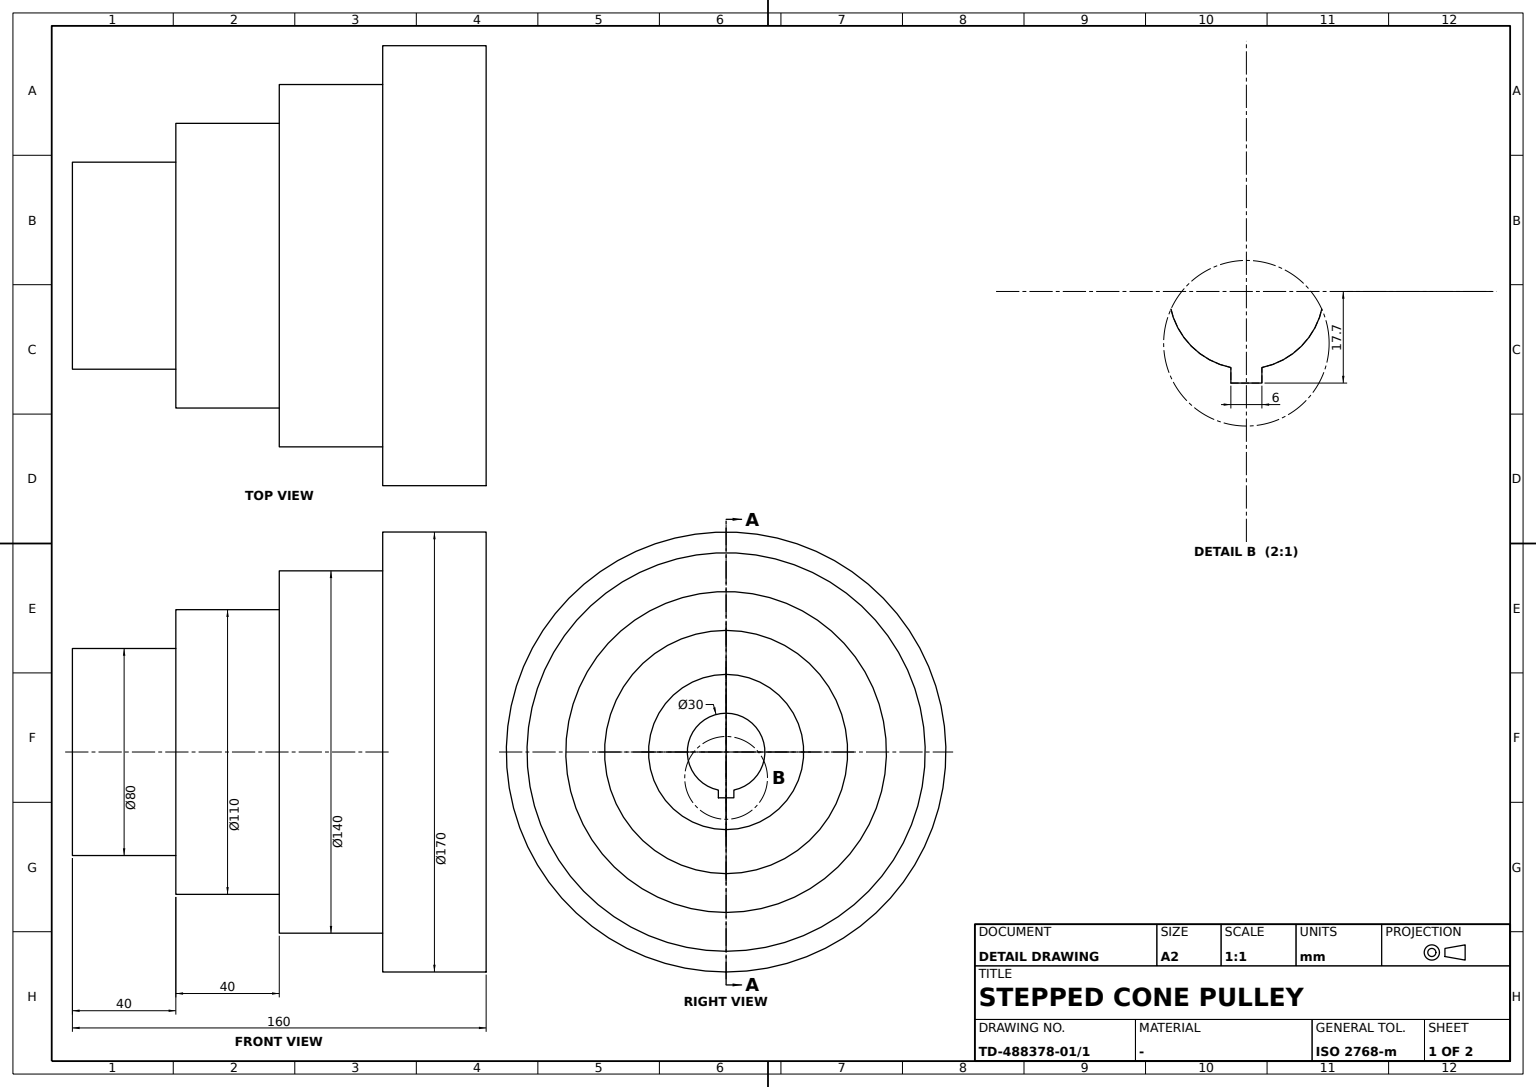
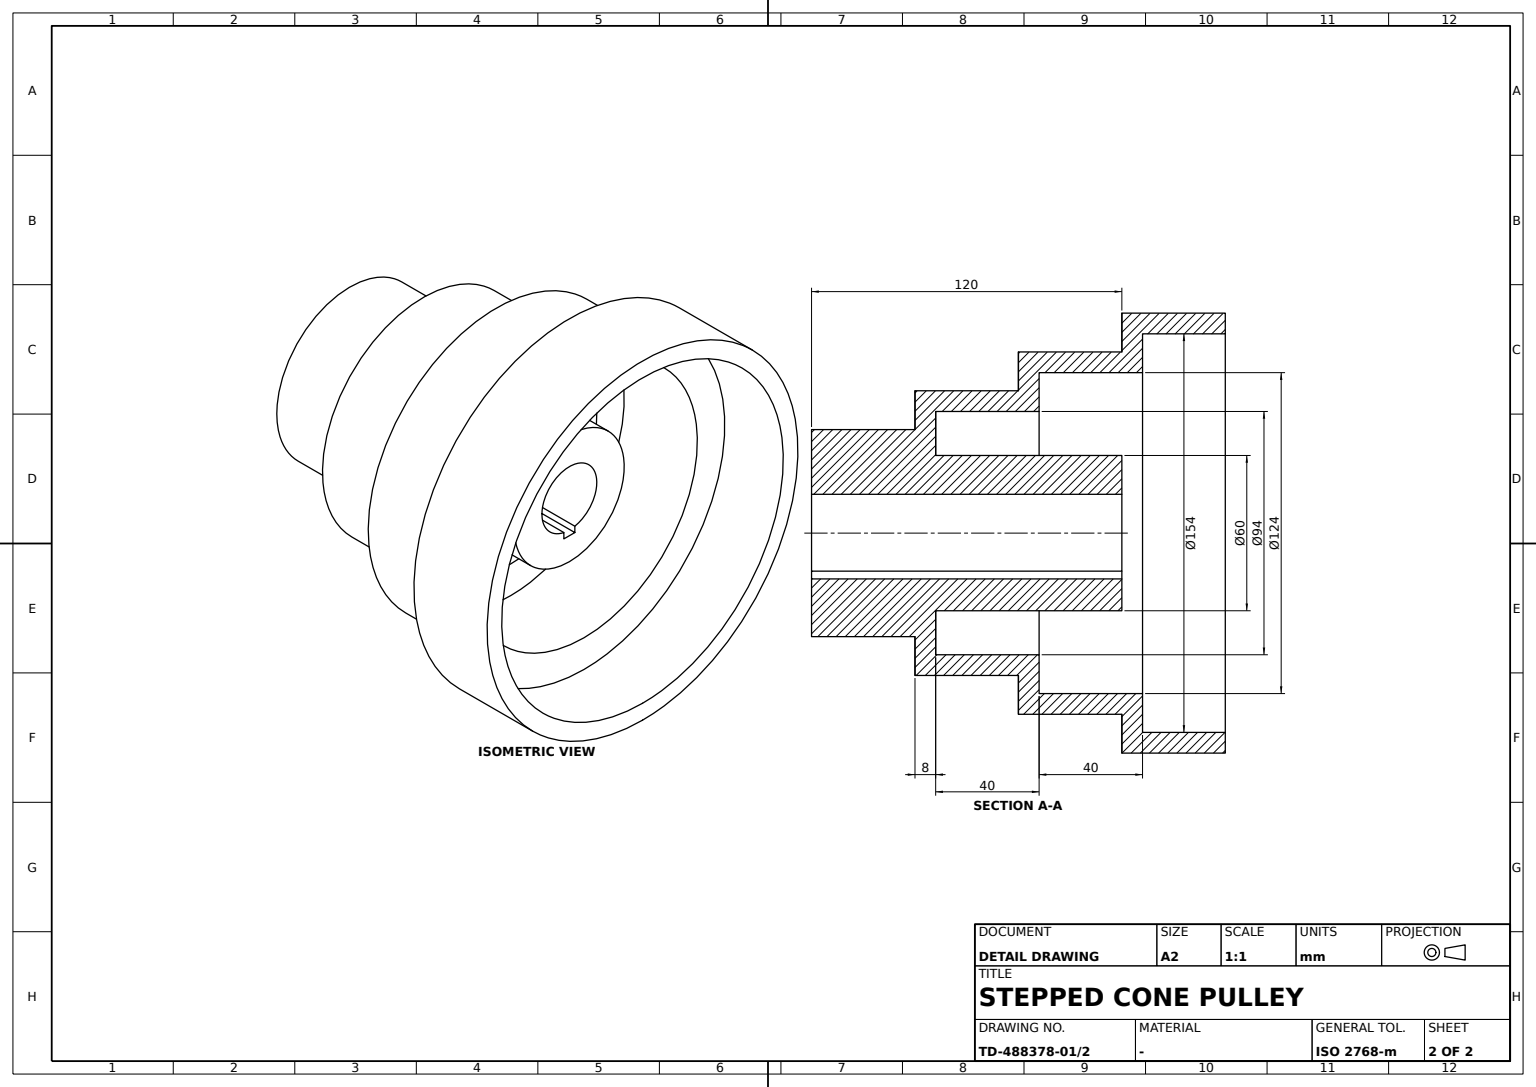
ISO-10303-21;
HEADER;
FILE_DESCRIPTION((''),'2;1');
FILE_NAME('','',(''),(''),'','','');
FILE_SCHEMA(('AUTOMOTIVE_DESIGN'));
ENDSEC;
DATA;
#1=APPLICATION_CONTEXT('');
#2=PRODUCT_CONTEXT('',#1,'mechanical');
#3=PRODUCT('','','',(#2));
#4=PRODUCT_DEFINITION_FORMATION('','',#3);
#5=PRODUCT_DEFINITION_CONTEXT('',#1,'design');
#6=PRODUCT_DEFINITION('','',#4,#5);
#7=PRODUCT_DEFINITION_SHAPE('','',#6);
#8=(LENGTH_UNIT()NAMED_UNIT(*)SI_UNIT(.MILLI.,.METRE.));
#9=(NAMED_UNIT(*)PLANE_ANGLE_UNIT()SI_UNIT($,.RADIAN.));
#10=(NAMED_UNIT(*)SI_UNIT($,.STERADIAN.)SOLID_ANGLE_UNIT());
#11=UNCERTAINTY_MEASURE_WITH_UNIT(LENGTH_MEASURE(0.005),#8,'distance_accuracy_value','');
#12=(GEOMETRIC_REPRESENTATION_CONTEXT(3)GLOBAL_UNCERTAINTY_ASSIGNED_CONTEXT((#11))GLOBAL_UNIT_ASSIGNED_CONTEXT((#8,#9,#10))REPRESENTATION_CONTEXT('',''));
#13=CARTESIAN_POINT('',(0.,80.,-70.));
#14=VERTEX_POINT('',#13);
#15=CARTESIAN_POINT('',(0.,80.,0.));
#16=DIRECTION('',(0.,-1.,0.));
#17=DIRECTION('',(0.,0.,-1.));
#18=AXIS2_PLACEMENT_3D('',#15,#16,#17);
#19=CIRCLE('',#18,70.);
#20=EDGE_CURVE('',#14,#14,#19,.T.);
#21=ORIENTED_EDGE('',*,*,#20,.T.);
#22=EDGE_LOOP('',(#21));
#23=FACE_BOUND('',#22,.T.);
#24=CARTESIAN_POINT('',(0.,80.,-55.));
#25=VERTEX_POINT('',#24);
#26=CIRCLE('',#18,55.);
#27=EDGE_CURVE('',#25,#25,#26,.T.);
#28=ORIENTED_EDGE('',*,*,#27,.F.);
#29=EDGE_LOOP('',(#28));
#30=FACE_BOUND('',#29,.T.);
#31=CARTESIAN_POINT('',(0.,80.,70.));
#32=DIRECTION('',(1.,0.,0.));
#33=AXIS2_PLACEMENT_3D('',#31,#16,#32);
#34=PLANE('',#33);
#35=ADVANCED_FACE('',(#23,#30),#34,.T.);
#36=CARTESIAN_POINT('',(0.,48.,-30.));
#37=VERTEX_POINT('',#36);
#38=CARTESIAN_POINT('',(0.,48.,0.));
#39=AXIS2_PLACEMENT_3D('',#38,#16,#17);
#40=CIRCLE('',#39,30.);
#41=EDGE_CURVE('',#37,#37,#40,.T.);
#42=ORIENTED_EDGE('',*,*,#41,.T.);
#43=EDGE_LOOP('',(#42));
#44=FACE_BOUND('',#43,.T.);
#45=CARTESIAN_POINT('',(0.,48.,-47.));
#46=VERTEX_POINT('',#45);
#47=CIRCLE('',#39,47.);
#48=EDGE_CURVE('',#46,#46,#47,.T.);
#49=ORIENTED_EDGE('',*,*,#48,.F.);
#50=EDGE_LOOP('',(#49));
#51=FACE_BOUND('',#50,.T.);
#52=CARTESIAN_POINT('',(0.,48.,30.));
#53=AXIS2_PLACEMENT_3D('',#52,#16,#32);
#54=PLANE('',#53);
#55=ADVANCED_FACE('',(#44,#51),#54,.F.);
#56=CARTESIAN_POINT('',(0.,160.,-85.));
#57=VERTEX_POINT('',#56);
#58=CARTESIAN_POINT('',(0.,160.,0.));
#59=AXIS2_PLACEMENT_3D('',#58,#16,#17);
#60=CIRCLE('',#59,85.);
#61=EDGE_CURVE('',#57,#57,#60,.T.);
#62=ORIENTED_EDGE('',*,*,#61,.F.);
#63=EDGE_LOOP('',(#62));
#64=FACE_BOUND('',#63,.T.);
#65=CARTESIAN_POINT('',(0.,160.,-77.));
#66=VERTEX_POINT('',#65);
#67=CIRCLE('',#59,77.);
#68=EDGE_CURVE('',#66,#66,#67,.T.);
#69=ORIENTED_EDGE('',*,*,#68,.T.);
#70=EDGE_LOOP('',(#69));
#71=FACE_BOUND('',#70,.T.);
#72=CARTESIAN_POINT('',(0.,160.,77.));
#73=AXIS2_PLACEMENT_3D('',#72,#16,#32);
#74=PLANE('',#73);
#75=ADVANCED_FACE('',(#64,#71),#74,.F.);
#76=CARTESIAN_POINT('',(3.,120.,-14.696938));
#77=VERTEX_POINT('',#76);
#78=CARTESIAN_POINT('',(3.,120.,-17.696938));
#79=VERTEX_POINT('',#78);
#80=VECTOR('',#17,1000.);
#81=LINE('',#76,#80);
#82=EDGE_CURVE('',#77,#79,#81,.T.);
#83=ORIENTED_EDGE('',*,*,#82,.F.);
#84=CARTESIAN_POINT('',(-3.,120.,-14.696938));
#85=VERTEX_POINT('',#84);
#86=CARTESIAN_POINT('',(0.,120.,0.));
#87=AXIS2_PLACEMENT_3D('',#86,#16,#17);
#88=CIRCLE('',#87,15.);
#89=EDGE_CURVE('',#77,#85,#88,.T.);
#90=ORIENTED_EDGE('',*,*,#89,.T.);
#91=CARTESIAN_POINT('',(-3.,120.,-17.696938));
#92=VERTEX_POINT('',#91);
#93=DIRECTION('',(0.,0.,1.));
#94=VECTOR('',#93,1000.);
#95=LINE('',#91,#94);
#96=EDGE_CURVE('',#92,#85,#95,.T.);
#97=ORIENTED_EDGE('',*,*,#96,.F.);
#98=DIRECTION('',(-1.,0.,0.));
#99=VECTOR('',#98,1000.);
#100=LINE('',#78,#99);
#101=EDGE_CURVE('',#79,#92,#100,.T.);
#102=ORIENTED_EDGE('',*,*,#101,.F.);
#103=EDGE_LOOP('',(#83,#90,#97,#102));
#104=FACE_BOUND('',#103,.T.);
#105=CARTESIAN_POINT('',(0.,120.,-30.));
#106=VERTEX_POINT('',#105);
#107=CIRCLE('',#87,30.);
#108=EDGE_CURVE('',#106,#106,#107,.T.);
#109=ORIENTED_EDGE('',*,*,#108,.F.);
#110=EDGE_LOOP('',(#109));
#111=FACE_BOUND('',#110,.T.);
#112=CARTESIAN_POINT('',(0.,120.,15.));
#113=AXIS2_PLACEMENT_3D('',#112,#16,#32);
#114=PLANE('',#113);
#115=ADVANCED_FACE('',(#104,#111),#114,.F.);
#116=CARTESIAN_POINT('',(0.,88.,-47.));
#117=VERTEX_POINT('',#116);
#118=CARTESIAN_POINT('',(0.,88.,0.));
#119=AXIS2_PLACEMENT_3D('',#118,#16,#17);
#120=CIRCLE('',#119,47.);
#121=EDGE_CURVE('',#117,#117,#120,.T.);
#122=ORIENTED_EDGE('',*,*,#121,.T.);
#123=EDGE_LOOP('',(#122));
#124=FACE_BOUND('',#123,.T.);
#125=CARTESIAN_POINT('',(0.,88.,-62.));
#126=VERTEX_POINT('',#125);
#127=CIRCLE('',#119,62.);
#128=EDGE_CURVE('',#126,#126,#127,.T.);
#129=ORIENTED_EDGE('',*,*,#128,.F.);
#130=EDGE_LOOP('',(#129));
#131=FACE_BOUND('',#130,.T.);
#132=CARTESIAN_POINT('',(0.,88.,47.));
#133=AXIS2_PLACEMENT_3D('',#132,#16,#32);
#134=PLANE('',#133);
#135=ADVANCED_FACE('',(#124,#131),#134,.F.);
#136=CARTESIAN_POINT('',(0.,40.,-40.));
#137=VERTEX_POINT('',#136);
#138=CARTESIAN_POINT('',(0.,40.,0.));
#139=AXIS2_PLACEMENT_3D('',#138,#16,#17);
#140=CIRCLE('',#139,40.);
#141=EDGE_CURVE('',#137,#137,#140,.T.);
#142=ORIENTED_EDGE('',*,*,#141,.T.);
#143=EDGE_LOOP('',(#142));
#144=FACE_BOUND('',#143,.T.);
#145=CARTESIAN_POINT('',(0.,0.,-40.));
#146=VERTEX_POINT('',#145);
#147=CARTESIAN_POINT('',(0.,0.,0.));
#148=AXIS2_PLACEMENT_3D('',#147,#16,#17);
#149=CIRCLE('',#148,40.);
#150=EDGE_CURVE('',#146,#146,#149,.T.);
#151=ORIENTED_EDGE('',*,*,#150,.F.);
#152=EDGE_LOOP('',(#151));
#153=FACE_BOUND('',#152,.T.);
#154=AXIS2_PLACEMENT_3D('',#15,#16,#32);
#155=CYLINDRICAL_SURFACE('',#154,40.);
#156=ADVANCED_FACE('',(#144,#153),#155,.T.);
#157=CARTESIAN_POINT('',(-3.,0.,-14.696938));
#158=VERTEX_POINT('',#157);
#159=VECTOR('',#16,1000.);
#160=LINE('',#157,#159);
#161=EDGE_CURVE('',#158,#85,#160,.F.);
#162=ORIENTED_EDGE('',*,*,#161,.F.);
#163=CARTESIAN_POINT('',(-3.,0.,-17.696938));
#164=VERTEX_POINT('',#163);
#165=LINE('',#163,#94);
#166=EDGE_CURVE('',#164,#158,#165,.T.);
#167=ORIENTED_EDGE('',*,*,#166,.F.);
#168=DIRECTION('',(0.,1.,0.));
#169=VECTOR('',#168,1000.);
#170=LINE('',#163,#169);
#171=EDGE_CURVE('',#164,#92,#170,.T.);
#172=ORIENTED_EDGE('',*,*,#171,.T.);
#173=ORIENTED_EDGE('',*,*,#96,.T.);
#174=EDGE_LOOP('',(#162,#167,#172,#173));
#175=FACE_BOUND('',#174,.T.);
#176=AXIS2_PLACEMENT_3D('',#163,#98,#93);
#177=PLANE('',#176);
#178=ADVANCED_FACE('',(#175),#177,.F.);
#179=ORIENTED_EDGE('',*,*,#82,.T.);
#180=CARTESIAN_POINT('',(3.,0.,-17.696938));
#181=VERTEX_POINT('',#180);
#182=LINE('',#180,#169);
#183=EDGE_CURVE('',#181,#79,#182,.T.);
#184=ORIENTED_EDGE('',*,*,#183,.F.);
#185=CARTESIAN_POINT('',(3.,0.,-14.696938));
#186=VERTEX_POINT('',#185);
#187=LINE('',#185,#80);
#188=EDGE_CURVE('',#186,#181,#187,.T.);
#189=ORIENTED_EDGE('',*,*,#188,.F.);
#190=LINE('',#185,#159);
#191=EDGE_CURVE('',#186,#77,#190,.F.);
#192=ORIENTED_EDGE('',*,*,#191,.T.);
#193=EDGE_LOOP('',(#179,#184,#189,#192));
#194=FACE_BOUND('',#193,.T.);
#195=AXIS2_PLACEMENT_3D('',#185,#32,#17);
#196=PLANE('',#195);
#197=ADVANCED_FACE('',(#194),#196,.F.);
#198=CARTESIAN_POINT('',(0.,128.,-77.));
#199=VERTEX_POINT('',#198);
#200=CARTESIAN_POINT('',(0.,128.,0.));
#201=AXIS2_PLACEMENT_3D('',#200,#16,#17);
#202=CIRCLE('',#201,77.);
#203=EDGE_CURVE('',#199,#199,#202,.T.);
#204=ORIENTED_EDGE('',*,*,#203,.T.);
#205=EDGE_LOOP('',(#204));
#206=FACE_BOUND('',#205,.T.);
#207=ORIENTED_EDGE('',*,*,#68,.F.);
#208=EDGE_LOOP('',(#207));
#209=FACE_BOUND('',#208,.T.);
#210=CYLINDRICAL_SURFACE('',#154,77.);
#211=ADVANCED_FACE('',(#206,#209),#210,.F.);
#212=ORIENTED_EDGE('',*,*,#128,.T.);
#213=EDGE_LOOP('',(#212));
#214=FACE_BOUND('',#213,.T.);
#215=CARTESIAN_POINT('',(0.,128.,-62.));
#216=VERTEX_POINT('',#215);
#217=CIRCLE('',#201,62.);
#218=EDGE_CURVE('',#216,#216,#217,.T.);
#219=ORIENTED_EDGE('',*,*,#218,.F.);
#220=EDGE_LOOP('',(#219));
#221=FACE_BOUND('',#220,.T.);
#222=CYLINDRICAL_SURFACE('',#154,62.);
#223=ADVANCED_FACE('',(#214,#221),#222,.F.);
#224=CARTESIAN_POINT('',(0.,40.,-55.));
#225=VERTEX_POINT('',#224);
#226=CIRCLE('',#139,55.);
#227=EDGE_CURVE('',#225,#225,#226,.T.);
#228=ORIENTED_EDGE('',*,*,#227,.T.);
#229=EDGE_LOOP('',(#228));
#230=FACE_BOUND('',#229,.T.);
#231=ORIENTED_EDGE('',*,*,#141,.F.);
#232=EDGE_LOOP('',(#231));
#233=FACE_BOUND('',#232,.T.);
#234=CARTESIAN_POINT('',(0.,40.,55.));
#235=AXIS2_PLACEMENT_3D('',#234,#16,#32);
#236=PLANE('',#235);
#237=ADVANCED_FACE('',(#230,#233),#236,.T.);
#238=ORIENTED_EDGE('',*,*,#61,.T.);
#239=EDGE_LOOP('',(#238));
#240=FACE_BOUND('',#239,.T.);
#241=CARTESIAN_POINT('',(0.,120.,-85.));
#242=VERTEX_POINT('',#241);
#243=CIRCLE('',#87,85.);
#244=EDGE_CURVE('',#242,#242,#243,.T.);
#245=ORIENTED_EDGE('',*,*,#244,.F.);
#246=EDGE_LOOP('',(#245));
#247=FACE_BOUND('',#246,.T.);
#248=CYLINDRICAL_SURFACE('',#154,85.);
#249=ADVANCED_FACE('',(#240,#247),#248,.T.);
#250=ORIENTED_EDGE('',*,*,#161,.T.);
#251=ORIENTED_EDGE('',*,*,#89,.F.);
#252=ORIENTED_EDGE('',*,*,#191,.F.);
#253=CIRCLE('',#148,15.);
#254=EDGE_CURVE('',#186,#158,#253,.T.);
#255=ORIENTED_EDGE('',*,*,#254,.T.);
#256=EDGE_LOOP('',(#250,#251,#252,#255));
#257=FACE_BOUND('',#256,.T.);
#258=CYLINDRICAL_SURFACE('',#154,15.);
#259=ADVANCED_FACE('',(#257),#258,.F.);
#260=ORIENTED_EDGE('',*,*,#227,.F.);
#261=EDGE_LOOP('',(#260));
#262=FACE_BOUND('',#261,.T.);
#263=ORIENTED_EDGE('',*,*,#27,.T.);
#264=EDGE_LOOP('',(#263));
#265=FACE_BOUND('',#264,.T.);
#266=CYLINDRICAL_SURFACE('',#154,55.);
#267=ADVANCED_FACE('',(#262,#265),#266,.T.);
#268=ORIENTED_EDGE('',*,*,#218,.T.);
#269=EDGE_LOOP('',(#268));
#270=FACE_BOUND('',#269,.T.);
#271=ORIENTED_EDGE('',*,*,#203,.F.);
#272=EDGE_LOOP('',(#271));
#273=FACE_BOUND('',#272,.T.);
#274=CARTESIAN_POINT('',(0.,128.,62.));
#275=AXIS2_PLACEMENT_3D('',#274,#16,#32);
#276=PLANE('',#275);
#277=ADVANCED_FACE('',(#270,#273),#276,.F.);
#278=ORIENTED_EDGE('',*,*,#101,.T.);
#279=ORIENTED_EDGE('',*,*,#171,.F.);
#280=LINE('',#180,#99);
#281=EDGE_CURVE('',#181,#164,#280,.T.);
#282=ORIENTED_EDGE('',*,*,#281,.F.);
#283=ORIENTED_EDGE('',*,*,#183,.T.);
#284=EDGE_LOOP('',(#278,#279,#282,#283));
#285=FACE_BOUND('',#284,.T.);
#286=AXIS2_PLACEMENT_3D('',#180,#17,#98);
#287=PLANE('',#286);
#288=ADVANCED_FACE('',(#285),#287,.F.);
#289=ORIENTED_EDGE('',*,*,#41,.F.);
#290=EDGE_LOOP('',(#289));
#291=FACE_BOUND('',#290,.T.);
#292=ORIENTED_EDGE('',*,*,#108,.T.);
#293=EDGE_LOOP('',(#292));
#294=FACE_BOUND('',#293,.T.);
#295=CYLINDRICAL_SURFACE('',#154,30.);
#296=ADVANCED_FACE('',(#291,#294),#295,.T.);
#297=CARTESIAN_POINT('',(0.,120.,-70.));
#298=VERTEX_POINT('',#297);
#299=CIRCLE('',#87,70.);
#300=EDGE_CURVE('',#298,#298,#299,.T.);
#301=ORIENTED_EDGE('',*,*,#300,.F.);
#302=EDGE_LOOP('',(#301));
#303=FACE_BOUND('',#302,.T.);
#304=ORIENTED_EDGE('',*,*,#244,.T.);
#305=EDGE_LOOP('',(#304));
#306=FACE_BOUND('',#305,.T.);
#307=ADVANCED_FACE('',(#303,#306),#114,.T.);
#308=ORIENTED_EDGE('',*,*,#20,.F.);
#309=EDGE_LOOP('',(#308));
#310=FACE_BOUND('',#309,.T.);
#311=ORIENTED_EDGE('',*,*,#300,.T.);
#312=EDGE_LOOP('',(#311));
#313=FACE_BOUND('',#312,.T.);
#314=CYLINDRICAL_SURFACE('',#154,70.);
#315=ADVANCED_FACE('',(#310,#313),#314,.T.);
#316=ORIENTED_EDGE('',*,*,#48,.T.);
#317=EDGE_LOOP('',(#316));
#318=FACE_BOUND('',#317,.T.);
#319=ORIENTED_EDGE('',*,*,#121,.F.);
#320=EDGE_LOOP('',(#319));
#321=FACE_BOUND('',#320,.T.);
#322=CYLINDRICAL_SURFACE('',#154,47.);
#323=ADVANCED_FACE('',(#318,#321),#322,.F.);
#324=ORIENTED_EDGE('',*,*,#166,.T.);
#325=ORIENTED_EDGE('',*,*,#254,.F.);
#326=ORIENTED_EDGE('',*,*,#188,.T.);
#327=ORIENTED_EDGE('',*,*,#281,.T.);
#328=EDGE_LOOP('',(#324,#325,#326,#327));
#329=FACE_BOUND('',#328,.T.);
#330=ORIENTED_EDGE('',*,*,#150,.T.);
#331=EDGE_LOOP('',(#330));
#332=FACE_BOUND('',#331,.T.);
#333=CARTESIAN_POINT('',(0.,0.,40.));
#334=AXIS2_PLACEMENT_3D('',#333,#16,#32);
#335=PLANE('',#334);
#336=ADVANCED_FACE('',(#329,#332),#335,.T.);
#337=CLOSED_SHELL('',(#35,#55,#75,#115,#135,#156,#178,#197,#211,#223,#237,#249,#259,#267,#277,#288,#296,#307,#315,#323,#336));
#338=MANIFOLD_SOLID_BREP('',#337);
#339=ADVANCED_BREP_SHAPE_REPRESENTATION('',(#338),#12);
#340=SHAPE_DEFINITION_REPRESENTATION(#7,#339);
ENDSEC;
END-ISO-10303-21;
